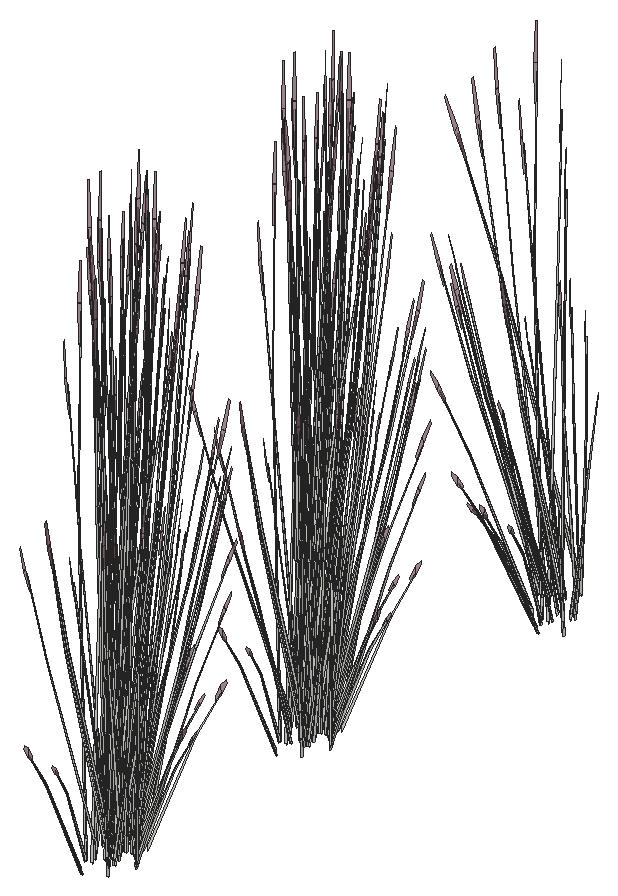
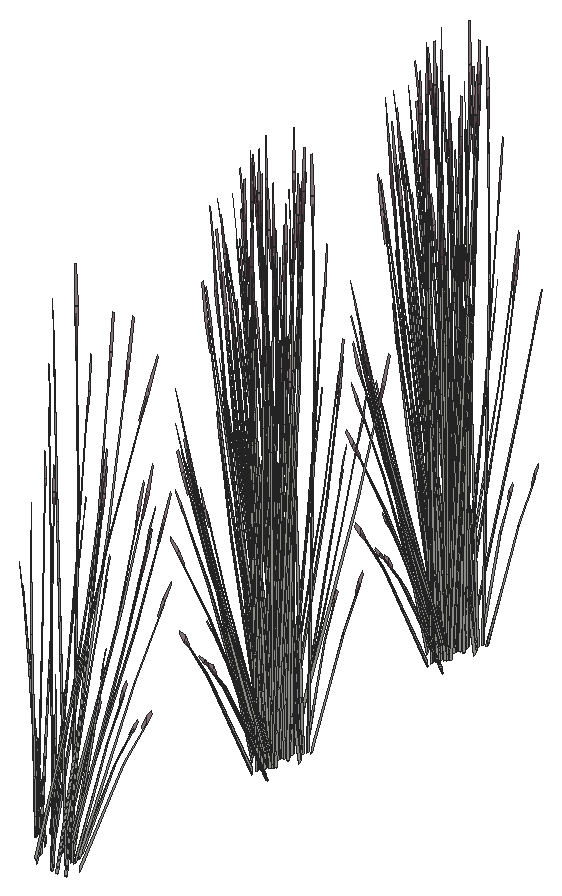
# SketchUp Ruby script. Lengths in inches.
U = 1.inch
M = Sketchup.active_model
def pt(a) = Geom::Point3d.new(a.map { |v| v * U })
def face(e, loops, mat)
  f = e.add_face(loops[0].map { |a| pt(a) })
  loops[1..].each { |l| e.add_face(l.map { |a| pt(a) }).erase! }
  f.material = f.back_material = mat if mat
  f
end
# faces: each face lists its corners as indices into pts; further lists are holes
def faces(e, pts, list, mat = nil) = list.each { |f| face(e, (f[0].is_a?(Array) ? f : [f]).map { |l| l.map { |i| pts[i] } }, mat) }
# xy, xz, yz: faces in a plane at the given z, y or x. An outline is a flat list of corners, or four numbers for a rectangle; further outlines are holes
def ring(l) = l.size == 4 ? [[l[0], l[1]], [l[2], l[1]], [l[2], l[3]], [l[0], l[3]]] : l.each_slice(2).to_a
def flat(e, list, mat, &to3) = list.each { |f| face(e, (f[0].is_a?(Array) ? f : [f]).map { |l| ring(l).map { |u, v| to3.(u, v) } }, mat) }
def xy(e, z, list, mat = nil) = flat(e, list, mat) { |x, y| [x, y, z] }
def xz(e, y, list, mat = nil) = flat(e, list, mat) { |x, z| [x, y, z] }
def yz(e, x, list, mat = nil) = flat(e, list, mat) { |y, z| [x, y, z] }
def lines(e, pts, list) = list.each { |a, b| e.add_line(pt(pts[a]), pt(pts[b])) }
# prism: a flat outline (further loops are holes) pulled along v
def prism(e, loops, v, mat = nil)
  f = face(e, loops, mat); d = Geom::Vector3d.new(v.map { |x| x * U })
  f.pushpull(f.normal.samedirection?(d) ? d.length : -d.length)
end
def box(e, o, s, mat = nil) = prism(e, [[o, [o[0] + s[0], o[1], o[2]], [o[0] + s[0], o[1] + s[1], o[2]], [o[0], o[1] + s[1], o[2]]]], [0, 0, s[2]], mat)
def at(x, y, z, deg = 0) = Geom::Transformation.translation(pt([x, y, z])) * Geom::Transformation.rotation(ORIGIN, Z_AXIS, deg.degrees)
def axes(o, x, y, z) = Geom::Transformation.new([*x, 0, *y, 0, *z, 0, *pt(o).to_a, 1])
def part(name) = M.definitions.add(name)
# library, detail: a bought-in or finely detailed component or shape, given as its bounding box
def library(name, o, s) = part(name).tap { |d| box(d.entities, o, s) }
def detail(e, o, s) = box(e.add_group.entities, o, s)
def put(e, d, t, mat = nil) = e.add_instance(d, t).tap { |i| i.material = mat if mat }
def group(e, t, mat = nil) = e.add_group.tap { |g| g.transformation = t; g.material = mat if mat }.entities
root = M.entities
M.materials.add("LightPink_Translucent").color = [144, 107, 117]
M.materials["LightPink_Translucent"].alpha = 0.75
c1 = part("blade")
p = [[2.15,0.21,22],[0,0.17,0],[0.09,0.45,0],[2.18,0.31,22],[2.29,0.31,22],[0.38,0.45,0],
  [2.48,0.24,33],[2.49,0.24,33],[2.48,0.22,33]]
faces(c1.entities,p,[[0,1,2,3],[4,5,2,3],[6,3,4,7],[8,0,3,6]])
c2 = part("seeds")
p = [[0.3,-0.1,1.38],[-0.01,-0.03,1.59],[-0.01,-0.03,0.03],[0.14,-0.07,-0.07],[0.29,-0.03,3],[0.15,0.01,3.11]]
faces(c2.entities,p,[[0,1,2,3],[1,0,4,5]],"LightPink_Translucent")
c3 = part("blade with seeds")
put(c3.entities,c1,at(0,0,0))
put(c3.entities,c2,axes([2.4,0.25,30.99],[1.5799,-0.05474,1.17369],[-0.12525,1.92788,0.29478],[-0.07173,-0.02425,1.56792]))
put(root,c3,axes([432.43,136.27,-0.72],[-0.06312,0.01988,1.51654],[-0.34903,-0.22379,-0.23168],[0.00586,-0.18666,0.25832]))
put(root,c3,axes([433.48,137.7,2.28],[0.00979,-0.51041,-0.61099],[0.4123,0.03428,0.07373],[0.04351,-0.21623,0.8643]))
put(root,c3,axes([432.77,136.88,1.89],[0.11344,-0.42434,-0.30456],[0.33096,0.12377,0.39319],[-0.03035,-0.17085,0.75234]))
put(root,c3,axes([432.83,135.98,0.38],[0.04827,0.32177,0.9878],[-0.26778,-0.17821,0.72577],[0.02882,-0.16476,0.21757]))
put(root,c3,axes([433.4,137.53,2.03],[-0.26937,-0.37076,-0.43945],[0.28456,-0.3247,-0.34039],[0.04099,-0.18838,0.84085]))
put(root,c3,axes([433.65,137.39,1.89],[0.2546,-0.29052,-0.30456],[0.24101,0.33173,0.39319],[0.03667,-0.16855,0.75234]))
put(root,c3,axes([433.97,137.22,-0.72],[-0.05632,-0.04347,1.51654],[-0.14467,-0.48565,-0.23168],[0.09759,-0.13179,0.25832]))
put(root,c3,axes([433.97,138.59,2.28],[0.19655,-0.43539,-0.61099],[0.34443,0.30942,0.07373],[0.11736,-0.15774,0.8643]))
put(root,c3,axes([431.84,137.32,0.04],[-0.23526,-0.55293,0],[0.3936,-0.30836,-0.44382],[0.08964,-0.07023,1.40792]))
put(root,c3,axes([433.96,138.38,2.03],[-0.09666,-0.50384,-0.43945],[0.36608,-0.08814,-0.34039],[0.10491,-0.13533,0.84085]))
put(root,c3,axes([432.16,137.23,-0.26],[0.35217,-0.2759,-0.427],[0.2105,0.49473,0],[0.08021,-0.06284,1.35453]))
put(root,c3,axes([434.25,138.1875,0.23],[-0.13443,-0.01634,1.22981],[-0.13772,-0.43844,-0.26449],[0.16514,-0.12403,0.52581]))
put(root,c3,axes([432.58,138.37,-0.23],[0.25345,-0.41475,-0.53624],[0.31485,0.37608,-0.14074],[0.10156,-0.10346,1.18365]))
put(root,c3,axes([434.41,137.38,0.38],[-0.12533,0.28089,0.9878],[-0.10773,-0.37739,0.72577],[0.10352,-0.09457,0.21757]))
put(root,c3,axes([434.23,138.4375,1.89],[0.32754,-0.07886,-0.30456],[0.08649,0.45081,0.39319],[0.09386,-0.12109,0.75234]))
put(root,c3,axes([432.14,139.09,-0.1],[0.18257,-0.49721,-0.38476],[0.37935,0.23929,0.18517],[0,-0.11462,1.23533]))
put(root,c3,axes([432.31,138.85,0.29],[-0.04385,-0.62963,-0.25022],[0.45669,-0.03807,-0.43002],[0.08042,-0.08387,1.37348]))
put(root,c3,axes([432.25,137.45,-0.26],[0.35106,0.13653,-0.26641],[-0.08839,0.48081,0.26641],[0.07077,-0.05545,1.19518]))
put(root,c3,axes([432.37,139.34,0.09],[0.42398,0.26744,0.20696],[-0.20405,0.55571,0.43002],[0,-0.1281,1.38067]))
put(root,c3,axes([432.23,138.97,0.34],[-0.40861,0.03406,0.38476],[-0.03695,-0.56543,-0.18517],[0.07315,-0.05731,1.23533]))
put(root,c3,axes([434.13,139.5,2.03],[0.10194,-0.50193,-0.43945],[0.34951,0.17204,-0.34039],[0.14072,-0.04602,0.84085]))
put(root,c3,axes([433.58,137.46,0.04],[0.23526,-0.55293,0],[0.3936,0.30836,-0.44382],[0.08964,0.07023,1.40792]))
put(root,c3,axes([432.22,139.17,0.03],[0.1636,0.61702,0.39349],[-0.46745,0.21456,0.15441],[0.00571,-0.11338,1.36617]))
put(root,c3,axes([434.5,139.64,-0.3],[-0.24235,0.06622,1.21762],[-0.03858,-0.5271,0.0697],[0.16974,-0.07978,0.69287]))
put(root,c3,axes([434.94,139.18,-0.06],[-0.23329,-0.35284,-0.05579],[0.2555,-0.3233,-0.25298],[0.0724,-0.02276,0.83441]))
put(root,c3,axes([432.8,139.22,-0.1],[0,-0.63847,0],[0.47052,0,0],[0,0,1.54332]))
put(root,c3,axes([433.375,137.75,0.13],[-0.35217,-0.2759,0.427],[0.2105,-0.49473,0],[0.08021,0.06284,1.35453]))
put(root,c3,axes([434.0625,139.69,2.28],[0.33065,-0.2437,-0.61099],[0.18427,0.50165,0.07373],[0.15976,-0.05699,0.8643]))
put(root,c3,axes([432.58,138.82,0.03],[-0.312,0.50076,0.39349],[-0.37066,-0.44204,0.15441],[0.07522,-0.04998,1.36617]))
put(root,c3,axes([432.92,139.72,-0.02],[-0.35001,-0.47494,-0.05273],[0.35022,-0.47523,0],[-0.01222,-0.01659,1.50991]))
put(root,c3,axes([432.04,138,0.13],[-0.1087,0.54839,0.15172],[-0.39778,-0.15519,0.30174],[0.06871,-0.00267,1.3795]))
put(root,c3,axes([431.875,138.4375,-0.63],[-0.37038,0.22092,1.10879],[-0.11789,-0.63387,0.43083],[0.22743,0.01055,1.26112]))
put(root,c3,axes([432.87,138.61,0.25],[0.07259,-0.49245,0.12452],[0.35466,0.08548,-0.35559],[0.06454,0.05057,1.09]))
put(root,c3,axes([434.77,139.3,-0.72],[-0.01967,-0.08377,1.51654],[0.1364,-0.49004,-0.23168],[0.13759,-0.00705,0.25832]))
put(root,c3,axes([432.72,138.74,0.34],[-0.22605,-0.46315,0.38476],[0.34239,-0.32614,-0.18517],[0.07315,0.05731,1.23533]))
put(root,c3,axes([432,140.82,0.13],[0.40434,-0.14646,0.15172],[0.09984,0.54504,0.30174],[-0.03606,-0.07941,1.3795]))
put(root,c3,axes([432.83,138.77,0.29],[0.37992,-0.36634,-0.25022],[0.25264,0.51764,-0.43002],[0.09374,0.05257,1.37348]))
put(root,c3,axes([434.34,139.73,1.89],[0.31272,0.15393,-0.30456],[-0.09121,0.44909,0.39319],[0.1259,-0.04118,0.75234]))
put(root,c3,axes([433.79,137.79,-0.26],[0.35217,0.2759,-0.427],[-0.2105,0.49473,0],[0.08021,0.06284,1.35453]))
put(root,c3,axes([433.12,139.37,-0.1],[0.42099,0,0],[0,0.57126,0],[0,0,1.5343]))
put(root,c3,axes([433.24,138.03,0.13],[-0.40434,0.14646,0.15172],[-0.09984,-0.54504,0.30174],[0.03606,0.07941,1.3795]))
put(root,c3,axes([433.69,138,-0.26],[0.08839,0.48081,-0.26641],[-0.35106,0.13653,0.26641],[0.07077,0.05545,1.19518]))
put(root,c3,axes([432.99,139.07,0.05],[-0.4756,-0.11626,0.42311],[0.09679,-0.6566,0.16603],[0.0695,0.0634,1.46899]))
put(root,c3,axes([432.61,140.7,-0.1],[-0.12277,-0.47573,0],[0.35059,-0.1666,0],[0,0,1.32759]))
put(root,c3,axes([433.07,140.63,-0.12],[0.39505,-0.18722,-0.1651],[0.13882,0.53931,0.00007],[0.04361,-0.02069,1.49552]))
put(root,c3,axes([433.2,140.85,0.13],[0.1087,-0.54839,0.15172],[0.39778,0.15519,0.30174],[-0.06871,0.00267,1.3795]))
put(root,c3,axes([433.11,139.61,-0.1],[0.26266,0.35642,0],[-0.26266,0.35642,0],[0,0,1.45569]))
put(root,c3,axes([433.82,139.46,0.13],[-0.29564,-0.40194,0.15172],[0.29793,-0.38985,0.30174],[-0.03265,0.08208,1.3795]))
put(root,c3,axes([433.28,138.85,-0.23],[0.39143,0.09047,-0.53624],[-0.0826,0.55804,-0.14074],[0.11681,0.06762,1.18365]))
put(root,c3,axes([435.01,139.82,0.38],[-0.23249,0.0911,0.9878],[0.10944,-0.37648,0.72577],[0.12334,0.02576,0.21757]))
put(root,c3,axes([432.52,140.91,-0.11],[-0.37935,-0.24773,0],[0.18257,-0.51475,0],[0,0,1.39928]))
put(root,c3,axes([433.11,139.19,0.34],[0.18257,-0.49721,0.38476],[0.37935,0.23929,-0.18517],[0,0.11462,1.23533]))
put(root,c3,axes([433.04,139.48,-0.03],[0,0.63816,-0.04848],[-0.47052,0,0],[0,0.02005,1.54256]))
put(root,c3,axes([433.07,139.03,-0.1],[0.22605,0.46315,-0.38476],[-0.34239,0.32614,0.18517],[0.07315,0.05731,1.23533]))
put(root,c3,axes([434.07,139.47,0.13],[0,-0.5518,0.427],[0.42099,0,0],[0,0.12568,1.35453]))
put(root,c3,axes([433.01,139.88,0.34],[0.40861,-0.03406,0.38476],[0.03695,0.56543,-0.18517],[-0.07315,0.05731,1.23533]))
put(root,c3,axes([433.27,139.31,0.25],[0.35059,-0.16092,0.12452],[0.12277,0.45952,-0.35559],[0,0.10113,1.09]))
put(root,c3,axes([434.57,140.43,0.23],[-0.09062,-0.13571,1.22981],[0.11791,-0.44895,-0.26449],[0.18335,0.06082,0.52581]))
put(root,c3,axes([432.95,140.92,-0.1],[0.37935,0.24773,0],[-0.18257,0.51475,0],[0,0,1.5046]))
put(root,c3,axes([433.02,140.125,0.25],[0.278,0.33153,0.12452],[-0.23189,0.37404,-0.35559],[-0.06454,0.05057,1.09]))
put(root,c3,axes([433.74,140.7,2.28],[0.37615,0.01329,-0.61099],[-0.02526,0.55946,0.07373],[0.15935,0.05904,0.8643]))
put(root,c3,axes([433.32,141.15,0.13],[0.35217,-0.2759,0.427],[0.2105,0.49473,0],[-0.08021,0.06284,1.35453]))
put(root,c3,axes([432.81,140.71,-0.03],[0.1636,0.63392,-0.05171],[-0.46745,0.22213,0],[0.00571,0.02214,1.48069]))
put(root,c3,axes([434.35,139.56,0.04],[0.47052,0,0],[0,0.61671,-0.44382],[0,0.14046,1.40792]))
put(root,c3,axes([434.17,139.88,-0.11],[-0.47029,-0.00441,-0.0428],[0,-0.61671,0.42951],[-0.01478,0.14039,1.36183]))
put(root,c3,axes([433.15,139.34,0.29],[0.42377,0.26329,-0.25022],[-0.20405,0.55571,-0.43002],[0.01332,0.13644,1.37348]))
put(root,c3,axes([433.97,140.93,1.89],[0.2141,0.34548,-0.30456],[-0.24447,0.32704,0.39319],[0.12421,0.04976,0.75234]))
put(root,c3,axes([434.07,139.97,-0.26],[-0.26266,0.34428,-0.26641],[-0.26266,-0.34428,0.26641],[0,0.11089,1.19518]))
put(root,c3,axes([433.1,139.76,-0.1],[-0.18257,0.49721,-0.38476],[-0.37935,-0.23929,0.18517],[0,0.11462,1.23533]))
put(root,c3,axes([433.11,141.18,0],[0.47108,0.17935,0.2645],[-0.11785,0.64108,-0.31383],[-0.07797,0.08023,1.41801]))
put(root,c3,axes([434.25,139.98,-0.26],[0,0.5518,-0.427],[-0.42099,0,0],[0,0.12568,1.35453]))
put(root,c3,axes([433.71,141.13,0.38],[-0.21187,-0.15866,0.9878],[0.27357,-0.16121,0.72577],[0.07379,0.13656,0.21757]))
put(root,c3,axes([433.4,141.53,0.04],[0.23526,0.55293,0],[-0.3936,0.30836,-0.44382],[-0.08964,0.07023,1.40792]))
put(root,c3,axes([433.77,141.72,-0.72],[0.02741,-0.07966,1.51654],[0.34514,-0.23462,-0.23168],[0.10464,0.12143,0.25832]))
put(root,c3,axes([433.32,139.91,-0.2],[0.13798,0.50522,-0.59522],[-0.39745,0.18195,-0.15622],[0.01525,0.17108,1.31385]))
put(root,c3,axes([433.24,141.35,2.03],[0.37131,-0.13117,-0.43945],[0.06495,0.49674,-0.34039],[0.09973,0.14235,0.84085]))
put(root,c3,axes([433.75,141.85,0.29],[-0.2413,-0.01731,0.90352],[0.15935,-0.36755,0.49885],[0.09532,0.13058,0.70873]))
put(root,c3,axes([432.96,140.96,0.23],[0.00664,-0.18292,1.22981],[0.31732,-0.20432,-0.26449],[0.09796,0.21893,0.52581]))
put(root,c3,axes([432.16,141.7,-0.72],[0.0609,-0.03003,1.51654],[0.36632,0.16527,-0.23168],[0.01071,0.18627,0.25832]))
put(root,c3,axes([432.41,141.58,2.03],[0.3699,0.13833,-0.43945],[-0.12679,0.47426,-0.34039],[0.03392,0.19095,0.84085]))
put(root,c3,axes([432.24,141.87,1.89],[-0.11344,0.42434,-0.30456],[-0.33096,-0.12377,0.39319],[0.03035,0.17085,0.75234]))
put(root,c3,axes([432.28,141.49,2.28],[0.17959,0.44867,-0.61099],[-0.36969,0.25004,0.07373],[0.042,0.21679,0.8643]))
put(root,c3,axes([433.22,158.72,0.23],[-0.10696,0.11169,1.22981],[-0.32033,-0.19549,-0.26449],[0.05938,-0.24312,0.52581]))
put(root,c3,axes([432.74,159.11,2.28],[-0.17959,-0.44867,-0.61099],[0.36969,-0.25004,0.07373],[-0.042,-0.21679,0.8643]))
put(root,c3,axes([432.43,158.12,-0.72],[-0.06312,0.01988,1.51654],[-0.34903,-0.22379,-0.23168],[0.00586,-0.18666,0.25832]))
put(root,c3,axes([433.48,159.55,2.28],[0.00979,-0.51041,-0.61099],[0.4123,0.03428,0.07373],[0.04351,-0.21623,0.8643]))
put(root,c3,axes([432.77,158.73,1.89],[0.11344,-0.42434,-0.30456],[0.33096,0.12377,0.39319],[-0.03035,-0.17085,0.75234]))
put(root,c3,axes([432.83,157.83,0.38],[0.04827,0.32177,0.9878],[-0.26778,-0.17821,0.72577],[0.02882,-0.16476,0.21757]))
put(root,c3,axes([433.4,159.38,2.03],[-0.26937,-0.37076,-0.43945],[0.28456,-0.3247,-0.34039],[0.04099,-0.18838,0.84085]))
put(root,c3,axes([433.65,159.24,1.89],[0.2546,-0.29052,-0.30456],[0.24101,0.33173,0.39319],[0.03667,-0.16855,0.75234]))
put(root,c3,axes([433.97,159.07,-0.72],[-0.05632,-0.04347,1.51654],[-0.14467,-0.48565,-0.23168],[0.09759,-0.13179,0.25832]))
put(root,c3,axes([433.97,160.4375,2.28],[0.19655,-0.43539,-0.61099],[0.34443,0.30942,0.07373],[0.11736,-0.15774,0.8643]))
put(root,c3,axes([431.84,159.17,0.04],[-0.23526,-0.55293,0],[0.3936,-0.30836,-0.44382],[0.08964,-0.07023,1.40792]))
put(root,c3,axes([433.96,160.23,2.03],[-0.09666,-0.50384,-0.43945],[0.36608,-0.08814,-0.34039],[0.10491,-0.13533,0.84085]))
put(root,c3,axes([432.16,159.08,-0.26],[0.35217,-0.2759,-0.427],[0.2105,0.49473,0],[0.08021,-0.06284,1.35453]))
put(root,c3,axes([434.25,160.04,0.23],[-0.13443,-0.01634,1.22981],[-0.13772,-0.43844,-0.26449],[0.16514,-0.12403,0.52581]))
put(root,c3,axes([432.58,160.22,-0.23],[0.25345,-0.41475,-0.53624],[0.31485,0.37608,-0.14074],[0.10156,-0.10346,1.18365]))
put(root,c3,axes([434.41,159.23,0.38],[-0.12533,0.28089,0.9878],[-0.10773,-0.37739,0.72577],[0.10352,-0.09457,0.21757]))
put(root,c3,axes([434.23,160.29,1.89],[0.32754,-0.07886,-0.30456],[0.08649,0.45081,0.39319],[0.09386,-0.12109,0.75234]))
put(root,c3,axes([432.14,160.94,-0.1],[0.18257,-0.49721,-0.38476],[0.37935,0.23929,0.18517],[0,-0.11462,1.23533]))
put(root,c3,axes([432.31,160.7,0.29],[-0.04385,-0.62963,-0.25022],[0.45669,-0.03807,-0.43002],[0.08042,-0.08387,1.37348]))
put(root,c3,axes([432.25,159.3,-0.26],[0.35106,0.13653,-0.26641],[-0.08839,0.48081,0.26641],[0.07077,-0.05545,1.19518]))
put(root,c3,axes([432.37,161.19,0.09],[0.42398,0.26744,0.20696],[-0.20405,0.55571,0.43002],[0,-0.1281,1.38067]))
put(root,c3,axes([432.23,160.82,0.34],[-0.40861,0.03406,0.38476],[-0.03695,-0.56543,-0.18517],[0.07315,-0.05731,1.23533]))
put(root,c3,axes([434.13,161.35,2.03],[0.10194,-0.50193,-0.43945],[0.34951,0.17204,-0.34039],[0.14072,-0.04602,0.84085]))
put(root,c3,axes([433.58,159.31,0.04],[0.23526,-0.55293,0],[0.3936,0.30836,-0.44382],[0.08964,0.07023,1.40792]))
put(root,c3,axes([432.22,161.02,0.03],[0.1636,0.61702,0.39349],[-0.46745,0.21456,0.15441],[0.00571,-0.11338,1.36617]))
put(root,c3,axes([434.5,161.49,-0.3],[-0.24235,0.06622,1.21762],[-0.03858,-0.5271,0.0697],[0.16974,-0.07978,0.69287]))
put(root,c3,axes([434.94,161.03,-0.06],[-0.23329,-0.35284,-0.05579],[0.2555,-0.3233,-0.25298],[0.0724,-0.02276,0.83441]))
put(root,c3,axes([432.8,161.07,-0.1],[0,-0.63847,0],[0.47052,0,0],[0,0,1.54332]))
put(root,c3,axes([433.375,159.6,0.13],[-0.35217,-0.2759,0.427],[0.2105,-0.49473,0],[0.08021,0.06284,1.35453]))
put(root,c3,axes([434.0625,161.54,2.28],[0.33065,-0.2437,-0.61099],[0.18427,0.50165,0.07373],[0.15976,-0.05699,0.8643]))
put(root,c3,axes([432.58,160.67,0.03],[-0.312,0.50076,0.39349],[-0.37066,-0.44204,0.15441],[0.07522,-0.04998,1.36617]))
put(root,c3,axes([432.92,161.57,-0.02],[-0.35001,-0.47494,-0.05273],[0.35022,-0.47523,0],[-0.01222,-0.01659,1.50991]))
put(root,c3,axes([432.04,159.85,0.13],[-0.1087,0.54839,0.15172],[-0.39778,-0.15519,0.30174],[0.06871,-0.00267,1.3795]))
put(root,c3,axes([431.875,160.29,-0.63],[-0.37038,0.22092,1.10879],[-0.11789,-0.63387,0.43083],[0.22743,0.01055,1.26112]))
put(root,c3,axes([432.87,160.46,0.25],[0.07259,-0.49245,0.12452],[0.35466,0.08548,-0.35559],[0.06454,0.05057,1.09]))
put(root,c3,axes([434.77,161.15,-0.72],[-0.01967,-0.08377,1.51654],[0.1364,-0.49004,-0.23168],[0.13759,-0.00705,0.25832]))
put(root,c3,axes([432.72,160.59,0.34],[-0.22605,-0.46315,0.38476],[0.34239,-0.32614,-0.18517],[0.07315,0.05731,1.23533]))
put(root,c3,axes([432,162.67,0.13],[0.40434,-0.14646,0.15172],[0.09984,0.54504,0.30174],[-0.03606,-0.07941,1.3795]))
put(root,c3,axes([432.83,160.62,0.29],[0.37992,-0.36634,-0.25022],[0.25264,0.51764,-0.43002],[0.09374,0.05257,1.37348]))
put(root,c3,axes([434.34,161.58,1.89],[0.31272,0.15393,-0.30456],[-0.09121,0.44909,0.39319],[0.1259,-0.04118,0.75234]))
put(root,c3,axes([433.79,159.64,-0.26],[0.35217,0.2759,-0.427],[-0.2105,0.49473,0],[0.08021,0.06284,1.35453]))
put(root,c3,axes([433.12,161.22,-0.1],[0.42099,0,0],[0,0.57126,0],[0,0,1.5343]))
put(root,c3,axes([433.24,159.875,0.13],[-0.40434,0.14646,0.15172],[-0.09984,-0.54504,0.30174],[0.03606,0.07941,1.3795]))
put(root,c3,axes([433.69,159.85,-0.26],[0.08839,0.48081,-0.26641],[-0.35106,0.13653,0.26641],[0.07077,0.05545,1.19518]))
put(root,c3,axes([432.99,160.93,0.05],[-0.4756,-0.11626,0.42311],[0.09679,-0.6566,0.16603],[0.0695,0.0634,1.46899]))
put(root,c3,axes([432.61,162.55,-0.1],[-0.12277,-0.47573,0],[0.35059,-0.1666,0],[0,0,1.32759]))
put(root,c3,axes([433.07,162.48,-0.12],[0.39505,-0.18722,-0.1651],[0.13882,0.53931,0.00007],[0.04361,-0.02069,1.49552]))
put(root,c3,axes([433.2,162.7,0.13],[0.1087,-0.54839,0.15172],[0.39778,0.15519,0.30174],[-0.06871,0.00267,1.3795]))
put(root,c3,axes([433.11,161.46,-0.1],[0.26266,0.35642,0],[-0.26266,0.35642,0],[0,0,1.45569]))
put(root,c3,axes([433.82,161.31,0.13],[-0.29564,-0.40194,0.15172],[0.29793,-0.38985,0.30174],[-0.03265,0.08208,1.3795]))
put(root,c3,axes([433.28,160.7,-0.23],[0.39143,0.09047,-0.53624],[-0.0826,0.55804,-0.14074],[0.11681,0.06762,1.18365]))
put(root,c3,axes([435.01,161.67,0.38],[-0.23249,0.0911,0.9878],[0.10944,-0.37648,0.72577],[0.12334,0.02576,0.21757]))
put(root,c3,axes([432.52,162.76,-0.11],[-0.37935,-0.24773,0],[0.18257,-0.51475,0],[0,0,1.39928]))
put(root,c3,axes([433.11,161.04,0.34],[0.18257,-0.49721,0.38476],[0.37935,0.23929,-0.18517],[0,0.11462,1.23533]))
put(root,c3,axes([433.04,161.33,-0.03],[0,0.63816,-0.04848],[-0.47052,0,0],[0,0.02005,1.54256]))
put(root,c3,axes([433.07,160.875,-0.1],[0.22605,0.46315,-0.38476],[-0.34239,0.32614,0.18517],[0.07315,0.05731,1.23533]))
put(root,c3,axes([434.07,161.32,0.13],[0,-0.5518,0.427],[0.42099,0,0],[0,0.12568,1.35453]))
put(root,c3,axes([433.01,161.73,0.34],[0.40861,-0.03406,0.38476],[0.03695,0.56543,-0.18517],[-0.07315,0.05731,1.23533]))
put(root,c3,axes([433.27,161.16,0.25],[0.35059,-0.16092,0.12452],[0.12277,0.45952,-0.35559],[0,0.10113,1.09]))
put(root,c3,axes([434.57,162.28,0.23],[-0.09062,-0.13571,1.22981],[0.11791,-0.44895,-0.26449],[0.18335,0.06082,0.52581]))
put(root,c3,axes([432.95,162.77,-0.1],[0.37935,0.24773,0],[-0.18257,0.51475,0],[0,0,1.5046]))
put(root,c3,axes([433.02,161.98,0.25],[0.278,0.33153,0.12452],[-0.23189,0.37404,-0.35559],[-0.06454,0.05057,1.09]))
put(root,c3,axes([433.74,162.55,2.28],[0.37615,0.01329,-0.61099],[-0.02526,0.55946,0.07373],[0.15935,0.05904,0.8643]))
put(root,c3,axes([433.32,163,0.13],[0.35217,-0.2759,0.427],[0.2105,0.49473,0],[-0.08021,0.06284,1.35453]))
put(root,c3,axes([432.81,162.5625,-0.03],[0.1636,0.63392,-0.05171],[-0.46745,0.22213,0],[0.00571,0.02214,1.48069]))
put(root,c3,axes([434.35,161.42,0.04],[0.47052,0,0],[0,0.61671,-0.44382],[0,0.14046,1.40792]))
put(root,c3,axes([434.17,161.73,-0.11],[-0.47029,-0.00441,-0.0428],[0,-0.61671,0.42951],[-0.01478,0.14039,1.36183]))
put(root,c3,axes([433.15,161.2,0.29],[0.42377,0.26329,-0.25022],[-0.20405,0.55571,-0.43002],[0.01332,0.13644,1.37348]))
put(root,c3,axes([433.97,162.78,1.89],[0.2141,0.34548,-0.30456],[-0.24447,0.32704,0.39319],[0.12421,0.04976,0.75234]))
put(root,c3,axes([434.07,161.82,-0.26],[-0.26266,0.34428,-0.26641],[-0.26266,-0.34428,0.26641],[0,0.11089,1.19518]))
put(root,c3,axes([433.1,161.61,-0.1],[-0.18257,0.49721,-0.38476],[-0.37935,-0.23929,0.18517],[0,0.11462,1.23533]))
put(root,c3,axes([433.11,163.03,0],[0.47108,0.17935,0.2645],[-0.11785,0.64108,-0.31383],[-0.07797,0.08023,1.41801]))
put(root,c3,axes([434.25,161.83,-0.26],[0,0.5518,-0.427],[-0.42099,0,0],[0,0.12568,1.35453]))
put(root,c3,axes([433.71,162.98,0.38],[-0.21187,-0.15866,0.9878],[0.27357,-0.16121,0.72577],[0.07379,0.13656,0.21757]))
put(root,c3,axes([433.4,163.38,0.04],[0.23526,0.55293,0],[-0.3936,0.30836,-0.44382],[-0.08964,0.07023,1.40792]))
put(root,c3,axes([433.77,163.57,-0.72],[0.02741,-0.07966,1.51654],[0.34514,-0.23462,-0.23168],[0.10464,0.12143,0.25832]))
put(root,c3,axes([433.32,161.76,-0.2],[0.13798,0.50522,-0.59522],[-0.39745,0.18195,-0.15622],[0.01525,0.17108,1.31385]))
put(root,c3,axes([433.24,163.2,2.03],[0.37131,-0.13117,-0.43945],[0.06495,0.49674,-0.34039],[0.09973,0.14235,0.84085]))
put(root,c3,axes([433.75,163.7,0.29],[-0.2413,-0.01731,0.90352],[0.15935,-0.36755,0.49885],[0.09532,0.13058,0.70873]))
put(root,c3,axes([432.96,162.81,0.23],[0.00664,-0.18292,1.22981],[0.31732,-0.20432,-0.26449],[0.09796,0.21893,0.52581]))
put(root,c3,axes([432.16,163.55,-0.72],[0.0609,-0.03003,1.51654],[0.36632,0.16527,-0.23168],[0.01071,0.18627,0.25832]))
put(root,c3,axes([432.41,163.43,2.03],[0.3699,0.13833,-0.43945],[-0.12679,0.47426,-0.34039],[0.03392,0.19095,0.84085]))
put(root,c3,axes([432.24,163.72,1.89],[-0.11344,0.42434,-0.30456],[-0.33096,-0.12377,0.39319],[0.03035,0.17085,0.75234]))
put(root,c3,axes([432.28,163.34,2.28],[0.17959,0.44867,-0.61099],[-0.36969,0.25004,0.07373],[0.042,0.21679,0.8643]))
put(root,c3,axes([436.68,183.82,0.23],[-0.10696,0.11169,1.22981],[-0.32033,-0.19549,-0.26449],[0.05938,-0.24312,0.52581]))
put(root,c3,axes([436.19,184.21,2.28],[-0.17959,-0.44867,-0.61099],[0.36969,-0.25004,0.07373],[-0.042,-0.21679,0.8643]))
put(root,c3,axes([435.02,183.61,0.23],[-0.02279,0.18051,1.22981],[-0.33311,0.15111,-0.26449],[-0.07787,-0.23331,0.52581]))
put(root,c3,axes([435.88,183.21,-0.72],[-0.06312,0.01988,1.51654],[-0.34903,-0.22379,-0.23168],[0.00586,-0.18666,0.25832]))
put(root,c3,axes([436.9375,184.65,2.28],[0.00979,-0.51041,-0.61099],[0.4123,0.03428,0.07373],[0.04351,-0.21623,0.8643]))
put(root,c3,axes([436.06,184.12,2.03],[-0.3699,-0.13833,-0.43945],[0.12679,-0.47426,-0.34039],[-0.03392,-0.19095,0.84085]))
put(root,c3,axes([436.28,182.93,0.38],[0.04827,0.32177,0.9878],[-0.26778,-0.17821,0.72577],[0.02882,-0.16476,0.21757]))
put(root,c3,axes([436.85,184.48,2.03],[-0.26937,-0.37076,-0.43945],[0.28456,-0.3247,-0.34039],[0.04099,-0.18838,0.84085]))
put(root,c3,axes([437.11,184.34,1.89],[0.2546,-0.29052,-0.30456],[0.24101,0.33173,0.39319],[0.03667,-0.16855,0.75234]))
put(root,c3,axes([434.91,183.32,0.38],[0.19628,0.19205,0.9878],[-0.28586,0.11545,0.72577],[-0.06116,-0.1476,0.21757]))
put(root,c3,axes([435.38,184.34,2.28],[-0.32086,-0.26671,-0.61099],[0.22803,-0.46737,0.07373],[-0.11625,-0.15925,0.8643]))
put(root,c3,axes([435.27,183.98,1.89],[-0.05812,-0.44446,-0.30456],[0.33222,-0.11736,0.39319],[-0.08923,-0.12737,0.75234]))
put(root,c3,axes([434.75,183.9,-0.72],[-0.03645,0.07269,1.51654],[-0.36835,0.15672,-0.23168],[-0.08898,-0.14257,0.25832]))
put(root,c3,axes([435.36,185.9,-0.2],[-0.15453,-0.56584,-0.60058],[0.44514,-0.20379,-0.15763],[-0.01708,-0.19161,1.32568]))
put(root,c3,axes([437.43,184.17,-0.72],[-0.05632,-0.04347,1.51654],[-0.14467,-0.48565,-0.23168],[0.09759,-0.13179,0.25832]))
put(root,c3,axes([435.23,184.35,2.03],[-0.37131,0.13117,-0.43945],[-0.06495,-0.49674,-0.34039],[-0.09973,-0.14235,0.84085]))
put(root,c3,axes([437.42,185.54,2.28],[0.19655,-0.43539,-0.61099],[0.34443,0.30942,0.07373],[0.11736,-0.15774,0.8643]))
put(root,c3,axes([435.3,184.27,0.04],[-0.23526,-0.55293,0],[0.3936,-0.30836,-0.44382],[0.08964,-0.07023,1.40792]))
put(root,c3,axes([437.41,185.33,2.03],[-0.09666,-0.50384,-0.43945],[0.36608,-0.08814,-0.34039],[0.10491,-0.13533,0.84085]))
put(root,c3,axes([435.82,183.6,-0.17],[-0.26003,0.31656,-0.03348],[-0.23826,-0.3467,-0.15179],[-0.01677,-0.09824,0.50065]))
put(root,c3,axes([436.15,187.35,0.86],[0.32517,0.22251,1.30084],[-0.31856,0.47936,0.51441],[-0.14269,-0.28411,1.09053]))
put(root,c3,axes([434.45,185.82,-0.26],[0,-0.5518,-0.427],[0.42099,0,0],[0,-0.12568,1.35453]))
put(root,c3,axes([435.62,184.18,-0.26],[0.35217,-0.2759,-0.427],[0.2105,0.49473,0],[0.08021,-0.06284,1.35453]))
put(root,c3,axes([437.71,185.14,0.23],[-0.13443,-0.01634,1.22981],[-0.13772,-0.43844,-0.26449],[0.16514,-0.12403,0.52581]))
put(root,c3,axes([436.04,185.31,-0.23],[0.25345,-0.41475,-0.53624],[0.31485,0.37608,-0.14074],[0.10156,-0.10346,1.18365]))
put(root,c3,axes([437.86,184.33,0.38],[-0.12533,0.28089,0.9878],[-0.10773,-0.37739,0.72577],[0.10352,-0.09457,0.21757]))
put(root,c3,axes([437.68,185.39,1.89],[0.32754,-0.07886,-0.30456],[0.08649,0.45081,0.39319],[0.09386,-0.12109,0.75234]))
put(root,c3,axes([435.59,186.04,-0.1],[0.18257,-0.49721,-0.38476],[0.37935,0.23929,0.18517],[0,-0.11462,1.23533]))
